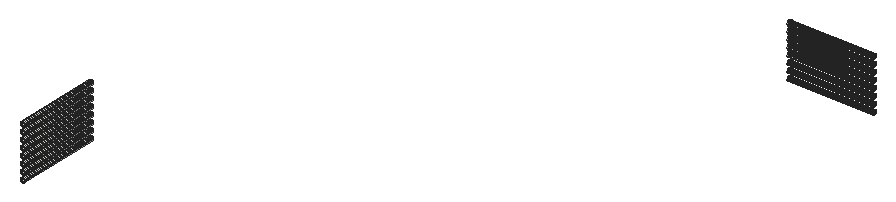
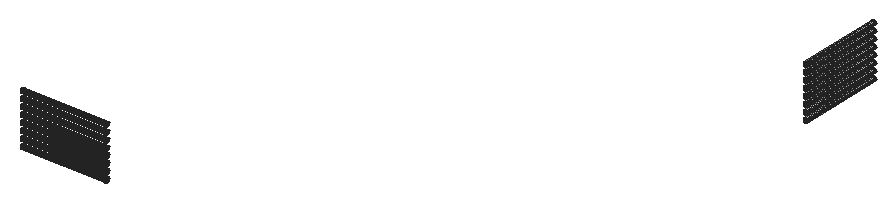
# SketchUp Ruby script. Lengths in inches.
U = 1.inch
M = Sketchup.active_model
def pt(a) = Geom::Point3d.new(a.map { |v| v * U })
def face(e, loops, mat)
  f = e.add_face(loops[0].map { |a| pt(a) })
  loops[1..].each { |l| e.add_face(l.map { |a| pt(a) }).erase! }
  f.material = f.back_material = mat if mat
  f
end
# faces: each face lists its corners as indices into pts; further lists are holes
def faces(e, pts, list, mat = nil) = list.each { |f| face(e, (f[0].is_a?(Array) ? f : [f]).map { |l| l.map { |i| pts[i] } }, mat) }
# xy, xz, yz: faces in a plane at the given z, y or x. An outline is a flat list of corners, or four numbers for a rectangle; further outlines are holes
def ring(l) = l.size == 4 ? [[l[0], l[1]], [l[2], l[1]], [l[2], l[3]], [l[0], l[3]]] : l.each_slice(2).to_a
def flat(e, list, mat, &to3) = list.each { |f| face(e, (f[0].is_a?(Array) ? f : [f]).map { |l| ring(l).map { |u, v| to3.(u, v) } }, mat) }
def xy(e, z, list, mat = nil) = flat(e, list, mat) { |x, y| [x, y, z] }
def xz(e, y, list, mat = nil) = flat(e, list, mat) { |x, z| [x, y, z] }
def yz(e, x, list, mat = nil) = flat(e, list, mat) { |y, z| [x, y, z] }
def lines(e, pts, list) = list.each { |a, b| e.add_line(pt(pts[a]), pt(pts[b])) }
# prism: a flat outline (further loops are holes) pulled along v
def prism(e, loops, v, mat = nil)
  f = face(e, loops, mat); d = Geom::Vector3d.new(v.map { |x| x * U })
  f.pushpull(f.normal.samedirection?(d) ? d.length : -d.length)
end
def box(e, o, s, mat = nil) = prism(e, [[o, [o[0] + s[0], o[1], o[2]], [o[0] + s[0], o[1] + s[1], o[2]], [o[0], o[1] + s[1], o[2]]]], [0, 0, s[2]], mat)
def at(x, y, z, deg = 0) = Geom::Transformation.translation(pt([x, y, z])) * Geom::Transformation.rotation(ORIGIN, Z_AXIS, deg.degrees)
def axes(o, x, y, z) = Geom::Transformation.new([*x, 0, *y, 0, *z, 0, *pt(o).to_a, 1])
def part(name) = M.definitions.add(name)
# library, detail: a bought-in or finely detailed component or shape, given as its bounding box
def library(name, o, s) = part(name).tap { |d| box(d.entities, o, s) }
def detail(e, o, s) = box(e.add_group.entities, o, s)
def put(e, d, t, mat = nil) = e.add_instance(d, t).tap { |i| i.material = mat if mat }
def group(e, t, mat = nil) = e.add_group.tap { |g| g.transformation = t; g.material = mat if mat }.entities
root = M.entities
p = [[83.53,662.8,1629.02],[82.57,662.8,1629.14],[82.57,806.17,1629.14],[83.53,806.17,1629.02],[84.48,662.8,1629.14],[84.48,806.17,1629.14],
  [697.99,1500.33,1629.14],[697.99,1501.28,1629.02],[841.36,1501.28,1629.02],[841.36,1500.33,1629.14],[697.99,1502.24,1629.14],[841.36,1502.24,1629.14],
  [81.68,662.8,1629.51],[81.68,806.17,1629.51],[85.37,662.8,1629.51],[85.37,806.17,1629.51],[697.99,1499.44,1629.51],[841.36,1499.44,1629.51],
  [697.99,1503.13,1629.51],[841.36,1503.13,1629.51],[80.92,662.8,1630.1],[80.92,806.17,1630.1],[86.13,662.8,1630.1],[86.13,806.17,1630.1],
  [697.99,1498.68,1630.1],[841.36,1498.68,1630.1],[697.99,1503.89,1630.1],[841.36,1503.89,1630.1],[80.33,662.8,1630.86],[80.33,806.17,1630.86],
  [86.72,662.8,1630.86],[86.72,806.17,1630.86],[697.99,1498.09,1630.86],[841.36,1498.09,1630.86],[697.99,1504.48,1630.86],[841.36,1504.48,1630.86],
  [79.97,662.8,1631.75],[79.97,806.17,1631.75],[87.09,662.8,1631.75],[87.09,806.17,1631.75],[697.99,1497.72,1631.75],[841.36,1497.72,1631.75],
  [697.99,1504.85,1631.75],[841.36,1504.85,1631.75],[79.84,662.8,1632.7],[79.84,806.17,1632.7],[87.21,662.8,1632.7],[87.21,806.17,1632.7],
  [697.99,1497.6,1632.7],[841.36,1497.6,1632.7],[697.99,1504.97,1632.7],[841.36,1504.97,1632.7],[79.97,662.8,1633.66],[79.97,806.17,1633.66],
  [87.09,662.8,1633.66],[87.09,806.17,1633.66],[697.99,1497.72,1633.66],[841.36,1497.72,1633.66],[697.99,1504.85,1633.66],[841.36,1504.85,1633.66],
  [80.33,662.8,1634.55],[80.33,806.17,1634.55],[86.72,662.8,1634.55],[86.72,806.17,1634.55],[697.99,1498.09,1634.55],[841.36,1498.09,1634.55],
  [697.99,1504.48,1634.55],[841.36,1504.48,1634.55],[80.92,662.8,1635.3125],[80.92,806.17,1635.3125],[86.13,662.8,1635.3125],[86.13,806.17,1635.3125],
  [697.99,1498.68,1635.3125],[841.36,1498.68,1635.3125],[697.99,1503.89,1635.3125],[841.36,1503.89,1635.3125],[81.68,662.8,1635.9],[81.68,806.17,1635.9],
  [85.37,662.8,1635.9],[85.37,806.17,1635.9],[697.99,1499.44,1635.9],[841.36,1499.44,1635.9],[697.99,1503.13,1635.9],[841.36,1503.13,1635.9],
  [82.57,662.8,1636.27],[82.57,806.17,1636.27],[84.48,662.8,1636.27],[84.48,806.17,1636.27],[697.99,1500.33,1636.27],[841.36,1500.33,1636.27],
  [697.99,1502.24,1636.27],[841.36,1502.24,1636.27],[83.53,662.8,1636.39],[83.53,806.17,1636.39],[697.99,1501.28,1636.39],[841.36,1501.28,1636.39],
  [83.53,662.8,1641.02],[82.57,662.8,1641.14],[82.57,806.17,1641.14],[83.53,806.17,1641.02],[84.48,662.8,1641.14],[84.48,806.17,1641.14],
  [697.99,1500.33,1641.14],[697.99,1501.28,1641.02],[841.36,1501.28,1641.02],[841.36,1500.33,1641.14],[697.99,1502.24,1641.14],[841.36,1502.24,1641.14],
  [81.68,662.8,1641.51],[81.68,806.17,1641.51],[85.37,662.8,1641.51],[85.37,806.17,1641.51],[697.99,1499.44,1641.51],[841.36,1499.44,1641.51],
  [697.99,1503.13,1641.51],[841.36,1503.13,1641.51],[80.92,662.8,1642.1],[80.92,806.17,1642.1],[86.13,662.8,1642.1],[86.13,806.17,1642.1],
  [697.99,1498.68,1642.1],[841.36,1498.68,1642.1],[697.99,1503.89,1642.1],[841.36,1503.89,1642.1],[80.33,662.8,1642.86],[80.33,806.17,1642.86],
  [86.72,662.8,1642.86],[86.72,806.17,1642.86],[697.99,1498.09,1642.86],[841.36,1498.09,1642.86],[697.99,1504.48,1642.86],[841.36,1504.48,1642.86],
  [79.97,662.8,1643.75],[79.97,806.17,1643.75],[87.09,662.8,1643.75],[87.09,806.17,1643.75],[697.99,1497.72,1643.75],[841.36,1497.72,1643.75],
  [697.99,1504.85,1643.75],[841.36,1504.85,1643.75],[79.84,662.8,1644.7],[79.84,806.17,1644.7],[87.21,662.8,1644.7],[87.21,806.17,1644.7],
  [697.99,1497.6,1644.7],[841.36,1497.6,1644.7],[697.99,1504.97,1644.7],[841.36,1504.97,1644.7],[79.97,662.8,1645.66],[79.97,806.17,1645.66],
  [87.09,662.8,1645.66],[87.09,806.17,1645.66],[697.99,1497.72,1645.66],[841.36,1497.72,1645.66],[697.99,1504.85,1645.66],[841.36,1504.85,1645.66],
  [80.33,662.8,1646.55],[80.33,806.17,1646.55],[86.72,662.8,1646.55],[86.72,806.17,1646.55],[697.99,1498.09,1646.55],[841.36,1498.09,1646.55],
  [697.99,1504.48,1646.55],[841.36,1504.48,1646.55],[80.92,662.8,1647.3125],[80.92,806.17,1647.3125],[86.13,662.8,1647.3125],[86.13,806.17,1647.3125],
  [697.99,1498.68,1647.3125],[841.36,1498.68,1647.3125],[697.99,1503.89,1647.3125],[841.36,1503.89,1647.3125],[81.68,662.8,1647.9],[81.68,806.17,1647.9],
  [85.37,662.8,1647.9],[85.37,806.17,1647.9],[697.99,1499.44,1647.9],[841.36,1499.44,1647.9],[697.99,1503.13,1647.9],[841.36,1503.13,1647.9],
  [82.57,662.8,1648.27],[82.57,806.17,1648.27],[84.48,662.8,1648.27],[84.48,806.17,1648.27],[697.99,1500.33,1648.27],[841.36,1500.33,1648.27],
  [697.99,1502.24,1648.27],[841.36,1502.24,1648.27],[83.53,662.8,1648.39],[83.53,806.17,1648.39],[697.99,1501.28,1648.39],[841.36,1501.28,1648.39],
  [83.53,662.8,1653.02],[82.57,662.8,1653.14],[82.57,806.17,1653.14],[83.53,806.17,1653.02],[84.48,662.8,1653.14],[84.48,806.17,1653.14],
  [697.99,1500.33,1653.14],[697.99,1501.28,1653.02],[841.36,1501.28,1653.02],[841.36,1500.33,1653.14],[697.99,1502.24,1653.14],[841.36,1502.24,1653.14],
  [81.68,662.8,1653.51],[81.68,806.17,1653.51],[85.37,662.8,1653.51],[85.37,806.17,1653.51],[697.99,1499.44,1653.51],[841.36,1499.44,1653.51],
  [697.99,1503.13,1653.51],[841.36,1503.13,1653.51],[80.92,662.8,1654.1],[80.92,806.17,1654.1],[86.13,662.8,1654.1],[86.13,806.17,1654.1],
  [697.99,1498.68,1654.1],[841.36,1498.68,1654.1],[697.99,1503.89,1654.1],[841.36,1503.89,1654.1],[80.33,662.8,1654.86],[80.33,806.17,1654.86],
  [86.72,662.8,1654.86],[86.72,806.17,1654.86],[697.99,1498.09,1654.86],[841.36,1498.09,1654.86],[697.99,1504.48,1654.86],[841.36,1504.48,1654.86],
  [79.97,662.8,1655.75],[79.97,806.17,1655.75],[87.09,662.8,1655.75],[87.09,806.17,1655.75],[697.99,1497.72,1655.75],[841.36,1497.72,1655.75],
  [697.99,1504.85,1655.75],[841.36,1504.85,1655.75],[79.84,662.8,1656.7],[79.84,806.17,1656.7],[87.21,662.8,1656.7],[87.21,806.17,1656.7],
  [697.99,1497.6,1656.7],[841.36,1497.6,1656.7],[697.99,1504.97,1656.7],[841.36,1504.97,1656.7],[79.97,662.8,1657.66],[79.97,806.17,1657.66],
  [87.09,662.8,1657.66],[87.09,806.17,1657.66],[697.99,1497.72,1657.66],[841.36,1497.72,1657.66],[697.99,1504.85,1657.66],[841.36,1504.85,1657.66],
  [80.33,662.8,1658.55],[80.33,806.17,1658.55],[86.72,662.8,1658.55],[86.72,806.17,1658.55],[697.99,1498.09,1658.55],[841.36,1498.09,1658.55],
  [697.99,1504.48,1658.55],[841.36,1504.48,1658.55],[80.92,662.8,1659.3125],[80.92,806.17,1659.3125],[86.13,662.8,1659.3125],[86.13,806.17,1659.3125],
  [697.99,1498.68,1659.3125],[841.36,1498.68,1659.3125],[697.99,1503.89,1659.3125],[841.36,1503.89,1659.3125],[81.68,662.8,1659.9],[81.68,806.17,1659.9],
  [85.37,662.8,1659.9],[85.37,806.17,1659.9],[697.99,1499.44,1659.9],[841.36,1499.44,1659.9],[697.99,1503.13,1659.9],[841.36,1503.13,1659.9],
  [82.57,662.8,1660.27],[82.57,806.17,1660.27],[84.48,662.8,1660.27],[84.48,806.17,1660.27],[697.99,1500.33,1660.27],[841.36,1500.33,1660.27],
  [697.99,1502.24,1660.27],[841.36,1502.24,1660.27],[83.53,662.8,1660.39],[83.53,806.17,1660.39],[697.99,1501.28,1660.39],[841.36,1501.28,1660.39],
  [83.53,662.8,1665.02],[82.57,662.8,1665.14],[82.57,806.17,1665.14],[83.53,806.17,1665.02],[84.48,662.8,1665.14],[84.48,806.17,1665.14],
  [697.99,1500.33,1665.14],[697.99,1501.28,1665.02],[841.36,1501.28,1665.02],[841.36,1500.33,1665.14],[697.99,1502.24,1665.14],[841.36,1502.24,1665.14],
  [81.68,662.8,1665.51],[81.68,806.17,1665.51],[85.37,662.8,1665.51],[85.37,806.17,1665.51],[697.99,1499.44,1665.51],[841.36,1499.44,1665.51],
  [697.99,1503.13,1665.51],[841.36,1503.13,1665.51],[80.92,662.8,1666.1],[80.92,806.17,1666.1],[86.13,662.8,1666.1],[86.13,806.17,1666.1],
  [697.99,1498.68,1666.1],[841.36,1498.68,1666.1],[697.99,1503.89,1666.1],[841.36,1503.89,1666.1],[80.33,662.8,1666.86],[80.33,806.17,1666.86],
  [86.72,662.8,1666.86],[86.72,806.17,1666.86],[697.99,1498.09,1666.86],[841.36,1498.09,1666.86],[697.99,1504.48,1666.86],[841.36,1504.48,1666.86],
  [79.97,662.8,1667.75],[79.97,806.17,1667.75],[87.09,662.8,1667.75],[87.09,806.17,1667.75],[697.99,1497.72,1667.75],[841.36,1497.72,1667.75],
  [697.99,1504.85,1667.75],[841.36,1504.85,1667.75],[79.84,662.8,1668.7],[79.84,806.17,1668.7],[87.21,662.8,1668.7],[87.21,806.17,1668.7],
  [697.99,1497.6,1668.7],[841.36,1497.6,1668.7],[697.99,1504.97,1668.7],[841.36,1504.97,1668.7],[79.97,662.8,1669.66],[79.97,806.17,1669.66],
  [87.09,662.8,1669.66],[87.09,806.17,1669.66],[697.99,1497.72,1669.66],[841.36,1497.72,1669.66],[697.99,1504.85,1669.66],[841.36,1504.85,1669.66],
  [80.33,662.8,1670.55],[80.33,806.17,1670.55],[86.72,662.8,1670.55],[86.72,806.17,1670.55],[697.99,1498.09,1670.55],[841.36,1498.09,1670.55],
  [697.99,1504.48,1670.55],[841.36,1504.48,1670.55],[80.92,662.8,1671.3125],[80.92,806.17,1671.3125],[86.13,662.8,1671.3125],[86.13,806.17,1671.3125],
  [697.99,1498.68,1671.3125],[841.36,1498.68,1671.3125],[697.99,1503.89,1671.3125],[841.36,1503.89,1671.3125],[81.68,662.8,1671.9],[81.68,806.17,1671.9],
  [85.37,662.8,1671.9],[85.37,806.17,1671.9],[697.99,1499.44,1671.9],[841.36,1499.44,1671.9],[697.99,1503.13,1671.9],[841.36,1503.13,1671.9],
  [82.57,662.8,1672.27],[82.57,806.17,1672.27],[84.48,662.8,1672.27],[84.48,806.17,1672.27],[697.99,1500.33,1672.27],[841.36,1500.33,1672.27],
  [697.99,1502.24,1672.27],[841.36,1502.24,1672.27],[83.53,662.8,1672.39],[83.53,806.17,1672.39],[697.99,1501.28,1672.39],[841.36,1501.28,1672.39],
  [83.53,662.8,1677.02],[82.57,662.8,1677.14],[82.57,806.17,1677.14],[83.53,806.17,1677.02],[84.48,662.8,1677.14],[84.48,806.17,1677.14],
  [697.99,1500.33,1677.14],[697.99,1501.28,1677.02],[841.36,1501.28,1677.02],[841.36,1500.33,1677.14],[697.99,1502.24,1677.14],[841.36,1502.24,1677.14],
  [81.68,662.8,1677.51],[81.68,806.17,1677.51],[85.37,662.8,1677.51],[85.37,806.17,1677.51],[697.99,1499.44,1677.51],[841.36,1499.44,1677.51],
  [697.99,1503.13,1677.51],[841.36,1503.13,1677.51],[80.92,662.8,1678.1],[80.92,806.17,1678.1],[86.13,662.8,1678.1],[86.13,806.17,1678.1],
  [697.99,1498.68,1678.1],[841.36,1498.68,1678.1],[697.99,1503.89,1678.1],[841.36,1503.89,1678.1],[80.33,662.8,1678.86],[80.33,806.17,1678.86],
  [86.72,662.8,1678.86],[86.72,806.17,1678.86],[697.99,1498.09,1678.86],[841.36,1498.09,1678.86],[697.99,1504.48,1678.86],[841.36,1504.48,1678.86],
  [79.97,662.8,1679.75],[79.97,806.17,1679.75],[87.09,662.8,1679.75],[87.09,806.17,1679.75],[697.99,1497.72,1679.75],[841.36,1497.72,1679.75],
  [697.99,1504.85,1679.75],[841.36,1504.85,1679.75],[79.84,662.8,1680.7],[79.84,806.17,1680.7],[87.21,662.8,1680.7],[87.21,806.17,1680.7],
  [697.99,1497.6,1680.7],[841.36,1497.6,1680.7],[697.99,1504.97,1680.7],[841.36,1504.97,1680.7],[79.97,662.8,1681.66],[79.97,806.17,1681.66],
  [87.09,662.8,1681.66],[87.09,806.17,1681.66],[697.99,1497.72,1681.66],[841.36,1497.72,1681.66],[697.99,1504.85,1681.66],[841.36,1504.85,1681.66],
  [80.33,662.8,1682.55],[80.33,806.17,1682.55],[86.72,662.8,1682.55],[86.72,806.17,1682.55],[697.99,1498.09,1682.55],[841.36,1498.09,1682.55],
  [697.99,1504.48,1682.55],[841.36,1504.48,1682.55],[80.92,662.8,1683.3125],[80.92,806.17,1683.3125],[86.13,662.8,1683.3125],[86.13,806.17,1683.3125],
  [697.99,1498.68,1683.3125],[841.36,1498.68,1683.3125],[697.99,1503.89,1683.3125],[841.36,1503.89,1683.3125],[81.68,662.8,1683.9],[81.68,806.17,1683.9],
  [85.37,662.8,1683.9],[85.37,806.17,1683.9],[697.99,1499.44,1683.9],[841.36,1499.44,1683.9],[697.99,1503.13,1683.9],[841.36,1503.13,1683.9],
  [82.57,662.8,1684.27],[82.57,806.17,1684.27],[84.48,662.8,1684.27],[84.48,806.17,1684.27],[697.99,1500.33,1684.27],[841.36,1500.33,1684.27],
  [697.99,1502.24,1684.27],[841.36,1502.24,1684.27],[83.53,662.8,1684.39],[83.53,806.17,1684.39],[697.99,1501.28,1684.39],[841.36,1501.28,1684.39],
  [83.53,662.8,1689.02],[82.57,662.8,1689.14],[82.57,806.17,1689.14],[83.53,806.17,1689.02],[84.48,662.8,1689.14],[84.48,806.17,1689.14],
  [697.99,1500.33,1689.14],[697.99,1501.28,1689.02],[841.36,1501.28,1689.02],[841.36,1500.33,1689.14],[697.99,1502.24,1689.14],[841.36,1502.24,1689.14],
  [81.68,662.8,1689.51],[81.68,806.17,1689.51],[85.37,662.8,1689.51],[85.37,806.17,1689.51],[697.99,1499.44,1689.51],[841.36,1499.44,1689.51],
  [697.99,1503.13,1689.51],[841.36,1503.13,1689.51],[80.92,662.8,1690.1],[80.92,806.17,1690.1],[86.13,662.8,1690.1],[86.13,806.17,1690.1],
  [697.99,1498.68,1690.1],[841.36,1498.68,1690.1],[697.99,1503.89,1690.1],[841.36,1503.89,1690.1],[80.33,662.8,1690.86],[80.33,806.17,1690.86],
  [86.72,662.8,1690.86],[86.72,806.17,1690.86],[697.99,1498.09,1690.86],[841.36,1498.09,1690.86],[697.99,1504.48,1690.86],[841.36,1504.48,1690.86],
  [79.97,662.8,1691.75],[79.97,806.17,1691.75],[87.09,662.8,1691.75],[87.09,806.17,1691.75],[697.99,1497.72,1691.75],[841.36,1497.72,1691.75],
  [697.99,1504.85,1691.75],[841.36,1504.85,1691.75],[79.84,662.8,1692.7],[79.84,806.17,1692.7],[87.21,662.8,1692.7],[87.21,806.17,1692.7],
  [697.99,1497.6,1692.7],[841.36,1497.6,1692.7],[697.99,1504.97,1692.7],[841.36,1504.97,1692.7],[79.97,662.8,1693.66],[79.97,806.17,1693.66],
  [87.09,662.8,1693.66],[87.09,806.17,1693.66],[697.99,1497.72,1693.66],[841.36,1497.72,1693.66],[697.99,1504.85,1693.66],[841.36,1504.85,1693.66],
  [80.33,662.8,1694.55],[80.33,806.17,1694.55],[86.72,662.8,1694.55],[86.72,806.17,1694.55],[697.99,1498.09,1694.55],[841.36,1498.09,1694.55],
  [697.99,1504.48,1694.55],[841.36,1504.48,1694.55],[80.92,662.8,1695.3125],[80.92,806.17,1695.3125],[86.13,662.8,1695.3125],[86.13,806.17,1695.3125],
  [697.99,1498.68,1695.3125],[841.36,1498.68,1695.3125],[697.99,1503.89,1695.3125],[841.36,1503.89,1695.3125],[81.68,662.8,1695.9],[81.68,806.17,1695.9],
  [85.37,662.8,1695.9],[85.37,806.17,1695.9],[697.99,1499.44,1695.9],[841.36,1499.44,1695.9],[697.99,1503.13,1695.9],[841.36,1503.13,1695.9],
  [82.57,662.8,1696.27],[82.57,806.17,1696.27],[84.48,662.8,1696.27],[84.48,806.17,1696.27],[697.99,1500.33,1696.27],[841.36,1500.33,1696.27],
  [697.99,1502.24,1696.27],[841.36,1502.24,1696.27],[83.53,662.8,1696.39],[83.53,806.17,1696.39],[697.99,1501.28,1696.39],[841.36,1501.28,1696.39],
  [83.53,662.8,1701.02],[82.57,662.8,1701.14],[82.57,806.17,1701.14],[83.53,806.17,1701.02],[84.48,662.8,1701.14],[84.48,806.17,1701.14],
  [697.99,1500.33,1701.14],[697.99,1501.28,1701.02],[841.36,1501.28,1701.02],[841.36,1500.33,1701.14],[697.99,1502.24,1701.14],[841.36,1502.24,1701.14],
  [81.68,662.8,1701.51],[81.68,806.17,1701.51],[85.37,662.8,1701.51],[85.37,806.17,1701.51],[697.99,1499.44,1701.51],[841.36,1499.44,1701.51],
  [697.99,1503.13,1701.51],[841.36,1503.13,1701.51],[80.92,662.8,1702.1],[80.92,806.17,1702.1],[86.13,662.8,1702.1],[86.13,806.17,1702.1],
  [697.99,1498.68,1702.1],[841.36,1498.68,1702.1],[697.99,1503.89,1702.1],[841.36,1503.89,1702.1],[80.33,662.8,1702.86],[80.33,806.17,1702.86],
  [86.72,662.8,1702.86],[86.72,806.17,1702.86],[697.99,1498.09,1702.86],[841.36,1498.09,1702.86],[697.99,1504.48,1702.86],[841.36,1504.48,1702.86],
  [79.97,662.8,1703.75],[79.97,806.17,1703.75],[87.09,662.8,1703.75],[87.09,806.17,1703.75],[697.99,1497.72,1703.75],[841.36,1497.72,1703.75],
  [697.99,1504.85,1703.75],[841.36,1504.85,1703.75],[79.84,662.8,1704.7],[79.84,806.17,1704.7],[87.21,662.8,1704.7],[87.21,806.17,1704.7],
  [697.99,1497.6,1704.7],[841.36,1497.6,1704.7],[697.99,1504.97,1704.7],[841.36,1504.97,1704.7],[79.97,662.8,1705.66],[79.97,806.17,1705.66],
  [87.09,662.8,1705.66],[87.09,806.17,1705.66],[697.99,1497.72,1705.66],[841.36,1497.72,1705.66],[697.99,1504.85,1705.66],[841.36,1504.85,1705.66],
  [80.33,662.8,1706.55],[80.33,806.17,1706.55],[86.72,662.8,1706.55],[86.72,806.17,1706.55],[697.99,1498.09,1706.55],[841.36,1498.09,1706.55],
  [697.99,1504.48,1706.55],[841.36,1504.48,1706.55],[80.92,662.8,1707.3125],[80.92,806.17,1707.3125],[86.13,662.8,1707.3125],[86.13,806.17,1707.3125],
  [697.99,1498.68,1707.3125],[841.36,1498.68,1707.3125],[697.99,1503.89,1707.3125],[841.36,1503.89,1707.3125],[81.68,662.8,1707.9],[81.68,806.17,1707.9],
  [85.37,662.8,1707.9],[85.37,806.17,1707.9],[697.99,1499.44,1707.9],[841.36,1499.44,1707.9],[697.99,1503.13,1707.9],[841.36,1503.13,1707.9],
  [82.57,662.8,1708.27],[82.57,806.17,1708.27],[84.48,662.8,1708.27],[84.48,806.17,1708.27],[697.99,1500.33,1708.27],[841.36,1500.33,1708.27],
  [697.99,1502.24,1708.27],[841.36,1502.24,1708.27],[83.53,662.8,1708.39],[83.53,806.17,1708.39],[697.99,1501.28,1708.39],[841.36,1501.28,1708.39],
  [83.53,662.8,1713.02],[82.57,662.8,1713.14],[82.57,806.17,1713.14],[83.53,806.17,1713.02],[84.48,662.8,1713.14],[84.48,806.17,1713.14],
  [697.99,1500.33,1713.14],[697.99,1501.28,1713.02],[841.36,1501.28,1713.02],[841.36,1500.33,1713.14],[697.99,1502.24,1713.14],[841.36,1502.24,1713.14],
  [81.68,662.8,1713.51],[81.68,806.17,1713.51],[85.37,662.8,1713.51],[85.37,806.17,1713.51],[697.99,1499.44,1713.51],[841.36,1499.44,1713.51],
  [697.99,1503.13,1713.51],[841.36,1503.13,1713.51],[80.92,662.8,1714.1],[80.92,806.17,1714.1],[86.13,662.8,1714.1],[86.13,806.17,1714.1],
  [697.99,1498.68,1714.1],[841.36,1498.68,1714.1],[697.99,1503.89,1714.1],[841.36,1503.89,1714.1],[80.33,662.8,1714.86],[80.33,806.17,1714.86],
  [86.72,662.8,1714.86],[86.72,806.17,1714.86],[697.99,1498.09,1714.86],[841.36,1498.09,1714.86],[697.99,1504.48,1714.86],[841.36,1504.48,1714.86],
  [79.97,662.8,1715.75],[79.97,806.17,1715.75],[87.09,662.8,1715.75],[87.09,806.17,1715.75],[697.99,1497.72,1715.75],[841.36,1497.72,1715.75],
  [697.99,1504.85,1715.75],[841.36,1504.85,1715.75],[79.84,662.8,1716.7],[79.84,806.17,1716.7],[87.21,662.8,1716.7],[87.21,806.17,1716.7],
  [697.99,1497.6,1716.7],[841.36,1497.6,1716.7],[697.99,1504.97,1716.7],[841.36,1504.97,1716.7],[79.97,662.8,1717.66],[79.97,806.17,1717.66],
  [87.09,662.8,1717.66],[87.09,806.17,1717.66],[697.99,1497.72,1717.66],[841.36,1497.72,1717.66],[697.99,1504.85,1717.66],[841.36,1504.85,1717.66],
  [80.33,662.8,1718.55],[80.33,806.17,1718.55],[86.72,662.8,1718.55],[86.72,806.17,1718.55],[697.99,1498.09,1718.55],[841.36,1498.09,1718.55],
  [697.99,1504.48,1718.55],[841.36,1504.48,1718.55],[80.92,662.8,1719.3125],[80.92,806.17,1719.3125],[86.13,662.8,1719.3125],[86.13,806.17,1719.3125],
  [697.99,1498.68,1719.3125],[841.36,1498.68,1719.3125],[697.99,1503.89,1719.3125],[841.36,1503.89,1719.3125],[81.68,662.8,1719.9],[81.68,806.17,1719.9],
  [85.37,662.8,1719.9],[85.37,806.17,1719.9],[697.99,1499.44,1719.9],[841.36,1499.44,1719.9],[697.99,1503.13,1719.9],[841.36,1503.13,1719.9],
  [82.57,662.8,1720.27],[82.57,806.17,1720.27],[84.48,662.8,1720.27],[84.48,806.17,1720.27],[697.99,1500.33,1720.27],[841.36,1500.33,1720.27],
  [697.99,1502.24,1720.27],[841.36,1502.24,1720.27],[83.53,662.8,1720.39],[83.53,806.17,1720.39],[697.99,1501.28,1720.39],[841.36,1501.28,1720.39]]
faces(root,p,[[0,1,2,3],[4,0,3,5],[6,7,8,9],[7,10,11,8],[1,12,13,2],[14,4,5,15],[16,6,9,17],[10,18,19,11],
  [12,20,21,13],[22,14,15,23],[24,16,17,25],[18,26,27,19],[20,28,29,21],[30,22,23,31],[32,24,25,33],[26,34,35,27],
  [28,36,37,29],[38,30,31,39],[40,32,33,41],[34,42,43,35],[36,44,45,37],[46,38,39,47],[48,40,41,49],[42,50,51,43],
  [44,52,53,45],[54,46,47,55],[56,48,49,57],[50,58,59,51],[52,60,61,53],[62,54,55,63],[64,56,57,65],[58,66,67,59],
  [60,68,69,61],[70,62,63,71],[72,64,65,73],[66,74,75,67],[68,76,77,69],[78,70,71,79],[80,72,73,81],[74,82,83,75],
  [76,84,85,77],[86,78,79,87],[88,80,81,89],[82,90,91,83],[84,92,93,85],[92,86,87,93],[94,88,89,95],[90,94,95,91],
  [96,97,98,99],[100,96,99,101],[102,103,104,105],[103,106,107,104],[97,108,109,98],[110,100,101,111],[112,102,105,113],[106,114,115,107],
  [108,116,117,109],[118,110,111,119],[120,112,113,121],[114,122,123,115],[116,124,125,117],[126,118,119,127],[128,120,121,129],[122,130,131,123],
  [124,132,133,125],[134,126,127,135],[136,128,129,137],[130,138,139,131],[132,140,141,133],[142,134,135,143],[144,136,137,145],[138,146,147,139],
  [140,148,149,141],[150,142,143,151],[152,144,145,153],[146,154,155,147],[148,156,157,149],[158,150,151,159],[160,152,153,161],[154,162,163,155],
  [156,164,165,157],[166,158,159,167],[168,160,161,169],[162,170,171,163],[164,172,173,165],[174,166,167,175],[176,168,169,177],[170,178,179,171],
  [172,180,181,173],[182,174,175,183],[184,176,177,185],[178,186,187,179],[180,188,189,181],[188,182,183,189],[190,184,185,191],[186,190,191,187],
  [192,193,194,195],[196,192,195,197],[198,199,200,201],[199,202,203,200],[193,204,205,194],[206,196,197,207],[208,198,201,209],[202,210,211,203],
  [204,212,213,205],[214,206,207,215],[216,208,209,217],[210,218,219,211],[212,220,221,213],[222,214,215,223],[224,216,217,225],[218,226,227,219],
  [220,228,229,221],[230,222,223,231],[232,224,225,233],[226,234,235,227],[228,236,237,229],[238,230,231,239],[240,232,233,241],[234,242,243,235],
  [236,244,245,237],[246,238,239,247],[248,240,241,249],[242,250,251,243],[244,252,253,245],[254,246,247,255],[256,248,249,257],[250,258,259,251],
  [252,260,261,253],[262,254,255,263],[264,256,257,265],[258,266,267,259],[260,268,269,261],[270,262,263,271],[272,264,265,273],[266,274,275,267],
  [268,276,277,269],[278,270,271,279],[280,272,273,281],[274,282,283,275],[276,284,285,277],[284,278,279,285],[286,280,281,287],[282,286,287,283],
  [288,289,290,291],[292,288,291,293],[294,295,296,297],[295,298,299,296],[289,300,301,290],[302,292,293,303],[304,294,297,305],[298,306,307,299],
  [300,308,309,301],[310,302,303,311],[312,304,305,313],[306,314,315,307],[308,316,317,309],[318,310,311,319],[320,312,313,321],[314,322,323,315],
  [316,324,325,317],[326,318,319,327],[328,320,321,329],[322,330,331,323],[324,332,333,325],[334,326,327,335],[336,328,329,337],[330,338,339,331],
  [332,340,341,333],[342,334,335,343],[344,336,337,345],[338,346,347,339],[340,348,349,341],[350,342,343,351],[352,344,345,353],[346,354,355,347],
  [348,356,357,349],[358,350,351,359],[360,352,353,361],[354,362,363,355],[356,364,365,357],[366,358,359,367],[368,360,361,369],[362,370,371,363],
  [364,372,373,365],[374,366,367,375],[376,368,369,377],[370,378,379,371],[372,380,381,373],[380,374,375,381],[382,376,377,383],[378,382,383,379],
  [384,385,386,387],[388,384,387,389],[390,391,392,393],[391,394,395,392],[385,396,397,386],[398,388,389,399],[400,390,393,401],[394,402,403,395],
  [396,404,405,397],[406,398,399,407],[408,400,401,409],[402,410,411,403],[404,412,413,405],[414,406,407,415],[416,408,409,417],[410,418,419,411],
  [412,420,421,413],[422,414,415,423],[424,416,417,425],[418,426,427,419],[420,428,429,421],[430,422,423,431],[432,424,425,433],[426,434,435,427],
  [428,436,437,429],[438,430,431,439],[440,432,433,441],[434,442,443,435],[436,444,445,437],[446,438,439,447],[448,440,441,449],[442,450,451,443],
  [444,452,453,445],[454,446,447,455],[456,448,449,457],[450,458,459,451],[452,460,461,453],[462,454,455,463],[464,456,457,465],[458,466,467,459],
  [460,468,469,461],[470,462,463,471],[472,464,465,473],[466,474,475,467],[468,476,477,469],[476,470,471,477],[478,472,473,479],[474,478,479,475],
  [480,481,482,483],[484,480,483,485],[486,487,488,489],[487,490,491,488],[481,492,493,482],[494,484,485,495],[496,486,489,497],[490,498,499,491],
  [492,500,501,493],[502,494,495,503],[504,496,497,505],[498,506,507,499],[500,508,509,501],[510,502,503,511],[512,504,505,513],[506,514,515,507],
  [508,516,517,509],[518,510,511,519],[520,512,513,521],[514,522,523,515],[516,524,525,517],[526,518,519,527],[528,520,521,529],[522,530,531,523],
  [524,532,533,525],[534,526,527,535],[536,528,529,537],[530,538,539,531],[532,540,541,533],[542,534,535,543],[544,536,537,545],[538,546,547,539],
  [540,548,549,541],[550,542,543,551],[552,544,545,553],[546,554,555,547],[548,556,557,549],[558,550,551,559],[560,552,553,561],[554,562,563,555],
  [556,564,565,557],[566,558,559,567],[568,560,561,569],[562,570,571,563],[564,572,573,565],[572,566,567,573],[574,568,569,575],[570,574,575,571],
  [576,577,578,579],[580,576,579,581],[582,583,584,585],[583,586,587,584],[577,588,589,578],[590,580,581,591],[592,582,585,593],[586,594,595,587],
  [588,596,597,589],[598,590,591,599],[600,592,593,601],[594,602,603,595],[596,604,605,597],[606,598,599,607],[608,600,601,609],[602,610,611,603],
  [604,612,613,605],[614,606,607,615],[616,608,609,617],[610,618,619,611],[612,620,621,613],[622,614,615,623],[624,616,617,625],[618,626,627,619],
  [620,628,629,621],[630,622,623,631],[632,624,625,633],[626,634,635,627],[628,636,637,629],[638,630,631,639],[640,632,633,641],[634,642,643,635],
  [636,644,645,637],[646,638,639,647],[648,640,641,649],[642,650,651,643],[644,652,653,645],[654,646,647,655],[656,648,649,657],[650,658,659,651],
  [652,660,661,653],[662,654,655,663],[664,656,657,665],[658,666,667,659],[660,668,669,661],[668,662,663,669],[670,664,665,671],[666,670,671,667],
  [672,673,674,675],[676,672,675,677],[678,679,680,681],[679,682,683,680],[673,684,685,674],[686,676,677,687],[688,678,681,689],[682,690,691,683],
  [684,692,693,685],[694,686,687,695],[696,688,689,697],[690,698,699,691],[692,700,701,693],[702,694,695,703],[704,696,697,705],[698,706,707,699],
  [700,708,709,701],[710,702,703,711],[712,704,705,713],[706,714,715,707],[708,716,717,709],[718,710,711,719],[720,712,713,721],[714,722,723,715],
  [716,724,725,717],[726,718,719,727],[728,720,721,729],[722,730,731,723],[724,732,733,725],[734,726,727,735],[736,728,729,737],[730,738,739,731],
  [732,740,741,733],[742,734,735,743],[744,736,737,745],[738,746,747,739],[740,748,749,741],[750,742,743,751],[752,744,745,753],[746,754,755,747],
  [748,756,757,749],[758,750,751,759],[760,752,753,761],[754,762,763,755],[756,764,765,757],[764,758,759,765],[766,760,761,767],[762,766,767,763]])
